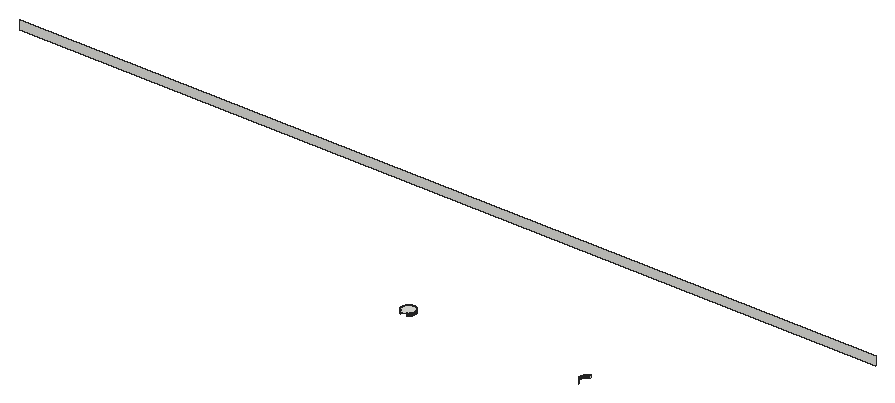
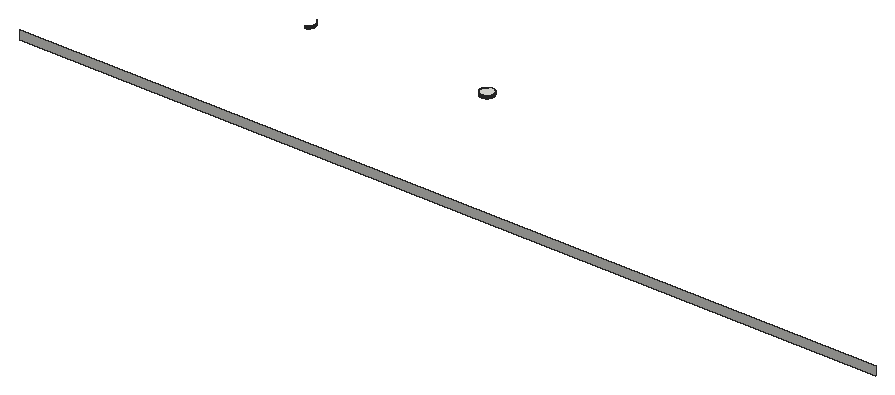
# SketchUp Ruby script. Lengths in inches.
U = 1.inch
M = Sketchup.active_model
def pt(a) = Geom::Point3d.new(a.map { |v| v * U })
def face(e, loops, mat)
  f = e.add_face(loops[0].map { |a| pt(a) })
  loops[1..].each { |l| e.add_face(l.map { |a| pt(a) }).erase! }
  f.material = f.back_material = mat if mat
  f
end
# faces: each face lists its corners as indices into pts; further lists are holes
def faces(e, pts, list, mat = nil) = list.each { |f| face(e, (f[0].is_a?(Array) ? f : [f]).map { |l| l.map { |i| pts[i] } }, mat) }
# xy, xz, yz: faces in a plane at the given z, y or x. An outline is a flat list of corners, or four numbers for a rectangle; further outlines are holes
def ring(l) = l.size == 4 ? [[l[0], l[1]], [l[2], l[1]], [l[2], l[3]], [l[0], l[3]]] : l.each_slice(2).to_a
def flat(e, list, mat, &to3) = list.each { |f| face(e, (f[0].is_a?(Array) ? f : [f]).map { |l| ring(l).map { |u, v| to3.(u, v) } }, mat) }
def xy(e, z, list, mat = nil) = flat(e, list, mat) { |x, y| [x, y, z] }
def xz(e, y, list, mat = nil) = flat(e, list, mat) { |x, z| [x, y, z] }
def yz(e, x, list, mat = nil) = flat(e, list, mat) { |y, z| [x, y, z] }
def lines(e, pts, list) = list.each { |a, b| e.add_line(pt(pts[a]), pt(pts[b])) }
# prism: a flat outline (further loops are holes) pulled along v
def prism(e, loops, v, mat = nil)
  f = face(e, loops, mat); d = Geom::Vector3d.new(v.map { |x| x * U })
  f.pushpull(f.normal.samedirection?(d) ? d.length : -d.length)
end
def box(e, o, s, mat = nil) = prism(e, [[o, [o[0] + s[0], o[1], o[2]], [o[0] + s[0], o[1] + s[1], o[2]], [o[0], o[1] + s[1], o[2]]]], [0, 0, s[2]], mat)
def at(x, y, z, deg = 0) = Geom::Transformation.translation(pt([x, y, z])) * Geom::Transformation.rotation(ORIGIN, Z_AXIS, deg.degrees)
def axes(o, x, y, z) = Geom::Transformation.new([*x, 0, *y, 0, *z, 0, *pt(o).to_a, 1])
def part(name) = M.definitions.add(name)
# library, detail: a bought-in or finely detailed component or shape, given as its bounding box
def library(name, o, s) = part(name).tap { |d| box(d.entities, o, s) }
def detail(e, o, s) = box(e.add_group.entities, o, s)
def put(e, d, t, mat = nil) = e.add_instance(d, t).tap { |i| i.material = mat if mat }
def group(e, t, mat = nil) = e.add_group.tap { |g| g.transformation = t; g.material = mat if mat }.entities
root = M.entities
xy(root,129,[[279.84,525,279.76,525.01,279.6875,525.02,279.61,525.03,279.45,525.05,279.375,525.07,279.3,525.08,279.22,525.1,279.15,525.125,279.07,525.15,279,525.17,278.92,525.2,278.71,525.29,278.64,525.33,278.57,525.36,278.43,525.44,278.37,525.48,278.3,525.53,278.24,525.57,278.17,525.62,277.93,525.82,277.88,525.88,277.82,525.93,277.62,526.17,277.57,526.24,277.53,526.3,277.48,526.37,277.44,526.43,277.36,526.57,277.33,526.64,277.29,526.71,277.2,526.92,277.17,527,277.15,527.07,277.125,527.15,277.1,527.22,277.08,527.3,277.07,527.375,277.05,527.45,277.03,527.61,277.02,527.6875,277.01,527.76,277,527.84,277,528.16,277.01,528.24,277.02,528.3125,277.03,528.39,277.05,528.55,277.07,528.625,277.08,528.7,277.1,528.78,277.125,528.85,277.15,528.93,277.17,529,277.2,529.08,277.29,529.29,277.33,529.36,277.36,529.43,277.44,529.57,277.48,529.63,277.53,529.7,277.57,529.76,277.62,529.83,277.82,530.07,277.88,530.12,277.93,530.18,278.17,530.38,278.24,530.43,278.3,530.47,278.37,530.52,278.43,530.56,278.57,530.64,278.64,530.67,278.71,530.71,278.92,530.8,279,530.83,279.07,530.85,279.15,530.875,279.22,530.9,279.3,530.92,279.375,530.93,279.45,530.95,279.61,530.97,279.6875,530.98,279.76,530.99,279.84,531,280.16,531,280.24,530.99,280.3125,530.98,280.39,530.97,280.55,530.95,280.625,530.93,280.7,530.92,280.78,530.9,280.85,530.875,280.93,530.85,281,530.83,281.08,530.8,281.29,530.71,281.36,530.67,281.43,530.64,281.57,530.56,281.63,530.52,281.7,530.47,281.76,530.43,281.83,530.38,282.07,530.18,282.12,530.12,282.18,530.07,282.38,529.83,282.43,529.76,282.47,529.7,282.52,529.63,282.56,529.57,282.64,529.43,282.67,529.36,282.71,529.29,282.8,529.08,282.83,529,282.85,528.93,282.875,528.85,282.9,528.78,282.92,528.7,282.93,528.625,282.95,528.55,282.97,528.39,282.98,528.3125,282.99,528.24,283,528.16,283,527.84,282.99,527.76,282.98,527.6875,282.97,527.61,282.95,527.45,282.93,527.375,282.92,527.3,282.9,527.22,282.875,527.15,282.85,527.07,282.83,527,282.8,526.92,282.71,526.71,282.67,526.64,282.64,526.57,282.56,526.43,282.52,526.37,282.47,526.3,282.43,526.24,282.38,526.17,282.18,525.93,282.12,525.88,282.07,525.82,281.83,525.62,281.76,525.57,281.7,525.53,281.63,525.48,281.57,525.44,281.43,525.36,281.36,525.33,281.29,525.29,281.08,525.2,281,525.17,280.93,525.15,280.85,525.125,280.78,525.1,280.7,525.08,280.625,525.07,280.55,525.05,280.39,525.03,280.3125,525.02,280.24,525.01,280.16,525]])
xz(root,531,[[279.84,128,279.92,129],[279.92,128,280,129],[280,128,280.08,129],[280.08,128,280.16,129]])
xz(root,600,[[48,128,432,132]])
yz(root,277,[[527.84,128,527.92,129],[527.92,128,528,129],[528,128,528.08,129],[528.08,128,528.16,129]])
yz(root,283,[[527.84,128,527.92,129],[527.92,128,528,129],[528,128,528.08,129],[528.08,128,528.16,129]])
yz(root,357,[[527.84,128,527.92,129],[527.92,128,528,129],[528,128,528.08,129],[528.08,128,528.16,129]])
p = [[278.64,525.33,128],[278.57,525.36,128],[278.57,525.36,129],[278.64,525.33,129],[281.43,525.36,128],[281.36,525.33,128],
  [281.36,525.33,129],[281.43,525.36,129],[358.64,525.33,128],[358.57,525.36,128],[358.57,525.36,129],[358.64,525.33,129],
  [278.5,525.4,128],[278.43,525.44,128],[278.43,525.44,129],[278.5,525.4,129],[278.37,525.48,128],[278.37,525.48,129],
  [281.5,525.4,128],[281.5,525.4,129],[281.57,525.44,128],[281.57,525.44,129],[281.63,525.48,128],[281.63,525.48,129],
  [358.5,525.4,128],[358.43,525.44,128],[358.43,525.44,129],[358.5,525.4,129],[358.37,525.48,128],[358.37,525.48,129],
  [278.3,525.53,128],[278.24,525.57,128],[278.24,525.57,129],[278.3,525.53,129],[281.7,525.53,128],[281.7,525.53,129],
  [281.76,525.57,128],[281.76,525.57,129],[358.3,525.53,128],[358.24,525.57,128],[358.24,525.57,129],[358.3,525.53,129],
  [278.17,525.62,128],[278.11,525.67,128],[278.11,525.67,129],[278.17,525.62,129],[281.83,525.62,128],[281.83,525.62,129],
  [281.89,525.67,128],[281.89,525.67,129],[358.17,525.62,128],[358.11,525.67,128],[358.11,525.67,129],[358.17,525.62,129],
  [278.05,525.72,128],[277.99,525.77,128],[277.99,525.77,129],[278.05,525.72,129],[281.95,525.72,128],[281.95,525.72,129],
  [282.01,525.77,128],[282.01,525.77,129],[358.05,525.72,128],[357.99,525.77,128],[357.99,525.77,129],[358.05,525.72,129],
  [277.93,525.82,128],[277.93,525.82,129],[277.88,525.88,128],[277.88,525.88,129],[282.07,525.82,128],[282.07,525.82,129],
  [282.12,525.88,128],[282.12,525.88,129],[357.93,525.82,128],[357.93,525.82,129],[357.88,525.88,128],[357.88,525.88,129],
  [277.82,525.93,128],[277.82,525.93,129],[277.77,525.99,128],[277.77,525.99,129],[282.18,525.93,128],[282.18,525.93,129],
  [282.23,525.99,128],[282.23,525.99,129],[357.82,525.93,128],[357.82,525.93,129],[357.77,525.99,128],[357.77,525.99,129],
  [277.72,526.05,128],[277.72,526.05,129],[282.28,526.05,128],[282.28,526.05,129],[357.72,526.05,128],[357.72,526.05,129],
  [277.67,526.11,128],[277.62,526.17,128],[277.62,526.17,129],[277.67,526.11,129],[282.33,526.11,128],[282.33,526.11,129],
  [282.38,526.17,128],[282.38,526.17,129],[357.67,526.11,128],[357.62,526.17,128],[357.62,526.17,129],[357.67,526.11,129],
  [277.57,526.24,128],[277.53,526.3,128],[277.53,526.3,129],[277.57,526.24,129],[282.43,526.24,128],[282.43,526.24,129],
  [282.47,526.3,128],[282.47,526.3,129],[357.57,526.24,128],[357.53,526.3,128],[357.53,526.3,129],[357.57,526.24,129],
  [277.48,526.37,128],[277.48,526.37,129],[282.52,526.37,128],[282.52,526.37,129],[357.48,526.37,128],[357.48,526.37,129],
  [277.44,526.43,128],[277.44,526.43,129],[277.4,526.5,128],[277.4,526.5,129],[282.56,526.43,128],[282.56,526.43,129],
  [282.6,526.5,128],[282.6,526.5,129],[357.44,526.43,128],[357.44,526.43,129],[357.4,526.5,128],[357.4,526.5,129],
  [277.36,526.57,128],[277.36,526.57,129],[282.64,526.57,128],[282.64,526.57,129],[357.36,526.57,128],[357.36,526.57,129],
  [277.33,526.64,128],[277.33,526.64,129],[277.29,526.71,128],[277.29,526.71,129],[282.67,526.64,128],[282.67,526.64,129],
  [282.71,526.71,128],[282.71,526.71,129],[357.33,526.64,128],[357.33,526.64,129],[357.29,526.71,128],[357.29,526.71,129],
  [277.26,526.78,128],[277.26,526.78,129],[282.74,526.78,128],[282.74,526.78,129],[357.26,526.78,128],[357.26,526.78,129],
  [277.23,526.85,128],[277.23,526.85,129],[282.77,526.85,128],[282.77,526.85,129],[357.23,526.85,128],[357.23,526.85,129],
  [277.2,526.92,128],[277.2,526.92,129],[277.17,527,128],[277.17,527,129],[282.8,526.92,128],[282.8,526.92,129],
  [282.83,527,128],[282.83,527,129],[357.2,526.92,128],[357.2,526.92,129],[357.17,527,128],[357.17,527,129],
  [277.15,527.07,128],[277.15,527.07,129],[282.85,527.07,128],[282.85,527.07,129],[357.15,527.07,128],[357.15,527.07,129],
  [277.125,527.15,128],[277.125,527.15,129],[277.1,527.22,128],[277.1,527.22,129],[282.875,527.15,128],[282.875,527.15,129],
  [282.9,527.22,128],[282.9,527.22,129],[357.125,527.15,128],[357.125,527.15,129],[357.1,527.22,128],[357.1,527.22,129],
  [277.08,527.3,128],[277.08,527.3,129],[282.92,527.3,128],[282.92,527.3,129],[357.08,527.3,128],[357.08,527.3,129],
  [277.07,527.375,128],[277.07,527.375,129],[282.93,527.375,128],[282.93,527.375,129],[357.07,527.375,128],[357.07,527.375,129],
  [277.05,527.45,128],[277.05,527.45,129],[282.95,527.45,128],[282.95,527.45,129],[357.05,527.45,128],[357.05,527.45,129],
  [277.04,527.53,128],[277.04,527.53,129],[277.03,527.61,128],[277.03,527.61,129],[282.96,527.53,128],[282.96,527.53,129],
  [282.97,527.61,128],[282.97,527.61,129],[357.04,527.53,128],[357.04,527.53,129],[357.03,527.61,128],[357.03,527.61,129],
  [277.02,527.6875,128],[277.02,527.6875,129],[282.98,527.6875,128],[282.98,527.6875,129],[357.02,527.6875,128],[357.02,527.6875,129],
  [277.01,527.76,128],[277.01,527.76,129],[282.99,527.76,128],[282.99,527.76,129],[357.01,527.76,128],[357.01,527.76,129],
  [277,527.84,128],[277,527.84,129],[283,527.84,128],[283,527.84,129],[357,527.84,128],[357,527.84,129],
  [277,528.16,128],[277.01,528.24,128],[277.01,528.24,129],[277,528.16,129],[277.02,528.3125,128],[277.02,528.3125,129],
  [282.99,528.24,128],[283,528.16,128],[283,528.16,129],[282.99,528.24,129],[282.98,528.3125,128],[282.98,528.3125,129],
  [357,528.16,128],[357.01,528.24,128],[357.01,528.24,129],[357,528.16,129],[357.02,528.3125,128],[357.02,528.3125,129],
  [277.03,528.39,128],[277.03,528.39,129],[282.97,528.39,128],[282.97,528.39,129],[357.03,528.39,128],[357.03,528.39,129],
  [277.04,528.47,128],[277.04,528.47,129],[282.96,528.47,128],[282.96,528.47,129],[357.04,528.47,128],[357.04,528.47,129],
  [277.05,528.55,128],[277.05,528.55,129],[277.07,528.625,128],[277.07,528.625,129],[282.95,528.55,128],[282.95,528.55,129],
  [282.93,528.625,128],[282.93,528.625,129],[357.05,528.55,128],[357.05,528.55,129],[357.07,528.625,128],[357.07,528.625,129],
  [277.08,528.7,128],[277.08,528.7,129],[282.92,528.7,128],[282.92,528.7,129],[357.08,528.7,128],[357.08,528.7,129],
  [277.1,528.78,128],[277.1,528.78,129],[282.9,528.78,128],[282.9,528.78,129],[357.1,528.78,128],[357.1,528.78,129],
  [277.125,528.85,128],[277.125,528.85,129],[282.875,528.85,128],[282.875,528.85,129],[357.125,528.85,128],[357.125,528.85,129],
  [277.15,528.93,128],[277.15,528.93,129],[277.17,529,128],[277.17,529,129],[282.83,529,128],[282.85,528.93,128],
  [282.85,528.93,129],[282.83,529,129],[357.15,528.93,128],[357.15,528.93,129],[357.17,529,128],[357.17,529,129],
  [277.2,529.08,128],[277.2,529.08,129],[282.8,529.08,128],[282.8,529.08,129],[357.2,529.08,128],[357.2,529.08,129],
  [277.23,529.15,128],[277.23,529.15,129],[277.26,529.22,128],[277.26,529.22,129],[282.74,529.22,128],[282.77,529.15,128],
  [282.77,529.15,129],[282.74,529.22,129],[357.23,529.15,128],[357.23,529.15,129],[357.26,529.22,128],[357.26,529.22,129],
  [277.29,529.29,128],[277.29,529.29,129],[282.71,529.29,128],[282.71,529.29,129],[357.29,529.29,128],[357.29,529.29,129],
  [277.33,529.36,128],[277.33,529.36,129],[282.67,529.36,128],[282.67,529.36,129],[357.33,529.36,128],[357.33,529.36,129],
  [277.36,529.43,128],[277.36,529.43,129],[277.4,529.5,128],[277.4,529.5,129],[282.64,529.43,128],[282.64,529.43,129],
  [282.6,529.5,128],[282.6,529.5,129],[357.36,529.43,128],[357.36,529.43,129],[357.4,529.5,128],[357.4,529.5,129],
  [277.44,529.57,128],[277.44,529.57,129],[282.56,529.57,128],[282.56,529.57,129],[357.44,529.57,128],[357.44,529.57,129],
  [277.48,529.63,128],[277.48,529.63,129],[277.53,529.7,128],[277.53,529.7,129],[282.52,529.63,128],[282.52,529.63,129],
  [282.47,529.7,128],[282.47,529.7,129],[357.48,529.63,128],[357.48,529.63,129],[357.53,529.7,128],[357.53,529.7,129],
  [277.57,529.76,128],[277.57,529.76,129],[282.43,529.76,128],[282.43,529.76,129],[357.57,529.76,128],[357.57,529.76,129],
  [277.62,529.83,128],[277.62,529.83,129],[277.67,529.89,128],[277.67,529.89,129],[282.33,529.89,128],[282.38,529.83,128],
  [282.38,529.83,129],[282.33,529.89,129],[357.62,529.83,128],[357.62,529.83,129],[357.67,529.89,128],[357.67,529.89,129],
  [277.72,529.95,128],[277.72,529.95,129],[277.77,530.01,128],[277.77,530.01,129],[282.23,530.01,128],[282.28,529.95,128],
  [282.28,529.95,129],[282.23,530.01,129],[357.72,529.95,128],[357.72,529.95,129],[357.77,530.01,128],[357.77,530.01,129],
  [277.82,530.07,128],[277.82,530.07,129],[282.18,530.07,128],[282.18,530.07,129],[357.82,530.07,128],[357.82,530.07,129],
  [277.88,530.12,128],[277.88,530.12,129],[277.93,530.18,128],[277.93,530.18,129],[282.12,530.12,128],[282.12,530.12,129],
  [282.07,530.18,128],[282.07,530.18,129],[357.88,530.12,128],[357.88,530.12,129],[357.93,530.18,128],[357.93,530.18,129],
  [277.99,530.23,128],[277.99,530.23,129],[278.05,530.28,128],[278.05,530.28,129],[281.95,530.28,128],[282.01,530.23,128],
  [282.01,530.23,129],[281.95,530.28,129],[357.99,530.23,128],[357.99,530.23,129],[358.05,530.28,128],[358.05,530.28,129],
  [278.11,530.33,128],[278.11,530.33,129],[278.17,530.38,128],[278.17,530.38,129],[281.83,530.38,128],[281.89,530.33,128],
  [281.89,530.33,129],[281.83,530.38,129],[358.11,530.33,128],[358.11,530.33,129],[358.17,530.38,128],[358.17,530.38,129],
  [278.24,530.43,128],[278.24,530.43,129],[278.3,530.47,128],[278.3,530.47,129],[281.7,530.47,128],[281.76,530.43,128],
  [281.76,530.43,129],[281.7,530.47,129],[358.24,530.43,128],[358.24,530.43,129],[358.3,530.47,128],[358.3,530.47,129],
  [278.37,530.52,128],[278.37,530.52,129],[278.43,530.56,128],[278.43,530.56,129],[281.63,530.52,128],[281.63,530.52,129],
  [281.57,530.56,128],[281.57,530.56,129],[358.37,530.52,128],[358.37,530.52,129],[358.43,530.56,128],[358.43,530.56,129],
  [278.5,530.6,128],[278.5,530.6,129],[278.57,530.64,128],[278.57,530.64,129],[278.64,530.67,128],[278.64,530.67,129],
  [281.43,530.64,128],[281.5,530.6,128],[281.5,530.6,129],[281.43,530.64,129],[281.36,530.67,128],[281.36,530.67,129],
  [358.5,530.6,128],[358.5,530.6,129],[358.57,530.64,128],[358.57,530.64,129],[358.64,530.67,128],[358.64,530.67,129],
  [278.71,530.71,128],[278.71,530.71,129],[278.78,530.74,128],[278.78,530.74,129],[278.85,530.77,128],[278.85,530.77,129],
  [281.15,530.77,128],[281.22,530.74,128],[281.22,530.74,129],[281.15,530.77,129],[281.29,530.71,128],[281.29,530.71,129],
  [358.71,530.71,128],[358.71,530.71,129],[358.78,530.74,128],[358.78,530.74,129],[358.85,530.77,128],[358.85,530.77,129],
  [278.92,530.8,128],[278.92,530.8,129],[279,530.83,128],[279,530.83,129],[279.07,530.85,128],[279.07,530.85,129],
  [280.93,530.85,128],[281,530.83,128],[281,530.83,129],[280.93,530.85,129],[281.08,530.8,128],[281.08,530.8,129],
  [358.92,530.8,128],[358.92,530.8,129],[359,530.83,128],[359,530.83,129],[359.07,530.85,128],[359.07,530.85,129],
  [279.15,530.875,128],[279.15,530.875,129],[279.22,530.9,128],[279.22,530.9,129],[279.3,530.92,128],[279.3,530.92,129],
  [279.375,530.93,128],[279.375,530.93,129],[279.45,530.95,128],[279.45,530.95,129],[279.53,530.96,128],[279.53,530.96,129],
  [280.55,530.95,128],[280.625,530.93,128],[280.625,530.93,129],[280.55,530.95,129],[280.47,530.96,128],[280.47,530.96,129],
  [280.7,530.92,128],[280.7,530.92,129],[280.78,530.9,128],[280.78,530.9,129],[280.85,530.875,128],[280.85,530.875,129],
  [359.15,530.875,128],[359.15,530.875,129],[359.22,530.9,128],[359.22,530.9,129],[359.3,530.92,128],[359.3,530.92,129],
  [279.61,530.97,128],[279.61,530.97,129],[279.6875,530.98,128],[279.6875,530.98,129],[279.76,530.99,128],[279.76,530.99,129],
  [279.84,531,128],[279.84,531,129],[280.24,530.99,128],[280.3125,530.98,128],[280.3125,530.98,129],[280.24,530.99,129],
  [280.16,531,128],[280.16,531,129],[280.39,530.97,128],[280.39,530.97,129]]
faces(root,p,[[0,1,2,3],[4,5,6,7],[8,9,10,11],[12,13,14,15],[13,16,17,14],[1,12,15,2],[18,4,7,19],[20,18,19,21],
  [22,20,21,23],[24,25,26,27],[25,28,29,26],[9,24,27,10],[30,31,32,33],[16,30,33,17],[34,22,23,35],[36,34,35,37],
  [38,39,40,41],[28,38,41,29],[42,43,44,45],[31,42,45,32],[46,36,37,47],[48,46,47,49],[50,51,52,53],[39,50,53,40],
  [54,55,56,57],[43,54,57,44],[58,48,49,59],[60,58,59,61],[62,63,64,65],[51,62,65,52],[55,66,67,56],[66,68,69,67],
  [70,60,61,71],[72,70,71,73],[63,74,75,64],[74,76,77,75],[68,78,79,69],[78,80,81,79],[82,72,73,83],[84,82,83,85],
  [76,86,87,77],[86,88,89,87],[80,90,91,81],[92,84,85,93],[88,94,95,89],[96,97,98,99],[90,96,99,91],[100,92,93,101],
  [102,100,101,103],[104,105,106,107],[94,104,107,95],[108,109,110,111],[97,108,111,98],[112,102,103,113],[114,112,113,115],[116,117,118,119],
  [105,116,119,106],[109,120,121,110],[122,114,115,123],[117,124,125,118],[120,126,127,121],[126,128,129,127],[130,122,123,131],[132,130,131,133],
  [124,134,135,125],[134,136,137,135],[128,138,139,129],[140,132,133,141],[136,142,143,137],[138,144,145,139],[144,146,147,145],[148,140,141,149],
  [150,148,149,151],[142,152,153,143],[152,154,155,153],[146,156,157,147],[158,150,151,159],[154,160,161,155],[156,162,163,157],[164,158,159,165],
  [160,166,167,161],[162,168,169,163],[168,170,171,169],[172,164,165,173],[174,172,173,175],[166,176,177,167],[176,178,179,177],[170,180,181,171],
  [182,174,175,183],[178,184,185,179],[180,186,187,181],[186,188,189,187],[190,182,183,191],[192,190,191,193],[184,194,195,185],[194,196,197,195],
  [188,198,199,189],[200,192,193,201],[196,202,203,197],[198,204,205,199],[206,200,201,207],[202,208,209,203],[204,210,211,205],[212,206,207,213],
  [208,214,215,209],[210,216,217,211],[216,218,219,217],[220,212,213,221],[222,220,221,223],[214,224,225,215],[224,226,227,225],[218,228,229,219],
  [230,222,223,231],[226,232,233,227],[228,234,235,229],[236,230,231,237],[232,238,239,233],[234,240,241,235],[242,236,237,243],[238,244,245,239],
  [246,247,248,249],[247,250,251,248],[252,253,254,255],[256,252,255,257],[258,259,260,261],[259,262,263,260],[250,264,265,251],[266,256,257,267],
  [262,268,269,263],[264,270,271,265],[272,266,267,273],[268,274,275,269],[270,276,277,271],[276,278,279,277],[280,272,273,281],[282,280,281,283],
  [274,284,285,275],[284,286,287,285],[278,288,289,279],[290,282,283,291],[286,292,293,287],[288,294,295,289],[296,290,291,297],[292,298,299,293],
  [294,300,301,295],[302,296,297,303],[298,304,305,299],[300,306,307,301],[306,308,309,307],[310,311,312,313],[311,302,303,312],[304,314,315,305],
  [314,316,317,315],[308,318,319,309],[320,310,313,321],[316,322,323,317],[318,324,325,319],[324,326,327,325],[328,329,330,331],[329,320,321,330],
  [322,332,333,323],[332,334,335,333],[326,336,337,327],[338,328,331,339],[334,340,341,335],[336,342,343,337],[344,338,339,345],[340,346,347,341],
  [342,348,349,343],[348,350,351,349],[352,344,345,353],[354,352,353,355],[346,356,357,347],[356,358,359,357],[350,360,361,351],[362,354,355,363],
  [358,364,365,359],[360,366,367,361],[366,368,369,367],[370,362,363,371],[372,370,371,373],[364,374,375,365],[374,376,377,375],[368,378,379,369],
  [380,372,373,381],[376,382,383,377],[378,384,385,379],[384,386,387,385],[388,389,390,391],[389,380,381,390],[382,392,393,383],[392,394,395,393],
  [386,396,397,387],[396,398,399,397],[400,401,402,403],[401,388,391,402],[394,404,405,395],[404,406,407,405],[398,408,409,399],[410,400,403,411],
  [406,412,413,407],[408,414,415,409],[414,416,417,415],[418,410,411,419],[420,418,419,421],[412,422,423,413],[422,424,425,423],[416,426,427,417],
  [426,428,429,427],[430,431,432,433],[431,420,421,432],[424,434,435,425],[434,436,437,435],[428,438,439,429],[438,440,441,439],[442,443,444,445],
  [443,430,433,444],[436,446,447,437],[446,448,449,447],[440,450,451,441],[450,452,453,451],[454,455,456,457],[455,442,445,456],[448,458,459,449],
  [458,460,461,459],[452,462,463,453],[462,464,465,463],[466,454,457,467],[468,466,467,469],[460,470,471,461],[470,472,473,471],[464,474,475,465],
  [474,476,477,475],[476,478,479,477],[480,481,482,483],[484,480,483,485],[481,468,469,482],[472,486,487,473],[486,488,489,487],[488,490,491,489],
  [478,492,493,479],[492,494,495,493],[494,496,497,495],[498,499,500,501],[499,502,503,500],[502,484,485,503],[490,504,505,491],[504,506,507,505],
  [506,508,509,507],[496,510,511,497],[510,512,513,511],[512,514,515,513],[516,517,518,519],[517,520,521,518],[520,498,501,521],[508,522,523,509],
  [522,524,525,523],[524,526,527,525],[514,528,529,515],[528,530,531,529],[530,532,533,531],[532,534,535,533],[534,536,537,535],[536,538,539,537],
  [540,541,542,543],[544,540,543,545],[541,546,547,542],[546,548,549,547],[548,550,551,549],[550,516,519,551],[526,552,553,527],[552,554,555,553],
  [554,556,557,555],[538,558,559,539],[558,560,561,559],[560,562,563,561],[562,564,565,563],[566,567,568,569],[570,566,569,571],[567,572,573,568],
  [572,544,545,573]])
